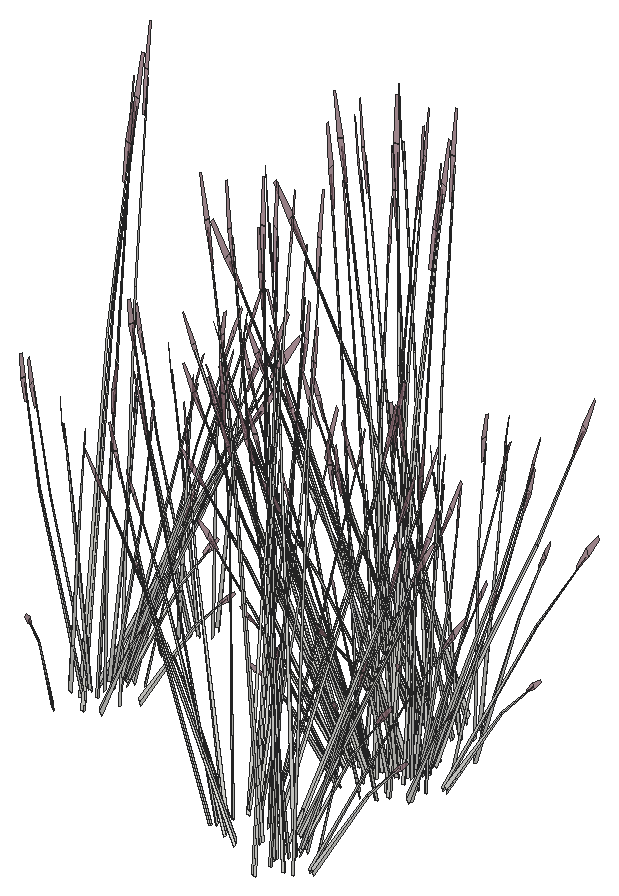
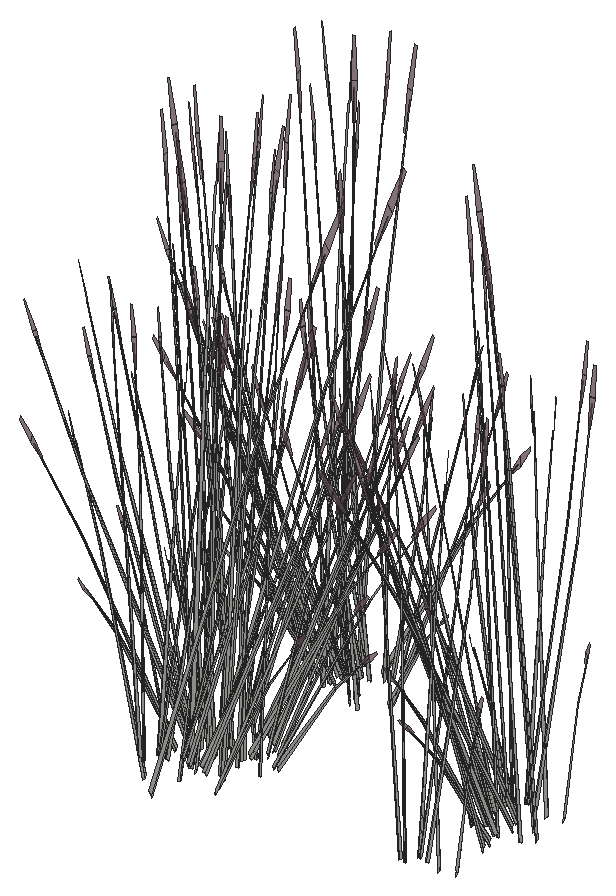
# SketchUp Ruby script. Lengths in inches.
U = 1.inch
M = Sketchup.active_model
def pt(a) = Geom::Point3d.new(a.map { |v| v * U })
def face(e, loops, mat)
  f = e.add_face(loops[0].map { |a| pt(a) })
  loops[1..].each { |l| e.add_face(l.map { |a| pt(a) }).erase! }
  f.material = f.back_material = mat if mat
  f
end
# faces: each face lists its corners as indices into pts; further lists are holes
def faces(e, pts, list, mat = nil) = list.each { |f| face(e, (f[0].is_a?(Array) ? f : [f]).map { |l| l.map { |i| pts[i] } }, mat) }
# xy, xz, yz: faces in a plane at the given z, y or x. An outline is a flat list of corners, or four numbers for a rectangle; further outlines are holes
def ring(l) = l.size == 4 ? [[l[0], l[1]], [l[2], l[1]], [l[2], l[3]], [l[0], l[3]]] : l.each_slice(2).to_a
def flat(e, list, mat, &to3) = list.each { |f| face(e, (f[0].is_a?(Array) ? f : [f]).map { |l| ring(l).map { |u, v| to3.(u, v) } }, mat) }
def xy(e, z, list, mat = nil) = flat(e, list, mat) { |x, y| [x, y, z] }
def xz(e, y, list, mat = nil) = flat(e, list, mat) { |x, z| [x, y, z] }
def yz(e, x, list, mat = nil) = flat(e, list, mat) { |y, z| [x, y, z] }
def lines(e, pts, list) = list.each { |a, b| e.add_line(pt(pts[a]), pt(pts[b])) }
# prism: a flat outline (further loops are holes) pulled along v
def prism(e, loops, v, mat = nil)
  f = face(e, loops, mat); d = Geom::Vector3d.new(v.map { |x| x * U })
  f.pushpull(f.normal.samedirection?(d) ? d.length : -d.length)
end
def box(e, o, s, mat = nil) = prism(e, [[o, [o[0] + s[0], o[1], o[2]], [o[0] + s[0], o[1] + s[1], o[2]], [o[0], o[1] + s[1], o[2]]]], [0, 0, s[2]], mat)
def at(x, y, z, deg = 0) = Geom::Transformation.translation(pt([x, y, z])) * Geom::Transformation.rotation(ORIGIN, Z_AXIS, deg.degrees)
def axes(o, x, y, z) = Geom::Transformation.new([*x, 0, *y, 0, *z, 0, *pt(o).to_a, 1])
def part(name) = M.definitions.add(name)
# library, detail: a bought-in or finely detailed component or shape, given as its bounding box
def library(name, o, s) = part(name).tap { |d| box(d.entities, o, s) }
def detail(e, o, s) = box(e.add_group.entities, o, s)
def put(e, d, t, mat = nil) = e.add_instance(d, t).tap { |i| i.material = mat if mat }
def group(e, t, mat = nil) = e.add_group.tap { |g| g.transformation = t; g.material = mat if mat }.entities
root = M.entities
M.materials.add("LightPink_Translucent").color = [144, 107, 117]
M.materials["LightPink_Translucent"].alpha = 0.75
c1 = part("blade")
p = [[2.15,0.21,22],[0,0.17,0],[0.09,0.45,0],[2.18,0.31,22],[2.29,0.31,22],[0.38,0.45,0],
  [2.48,0.24,33],[2.49,0.24,33],[2.48,0.22,33]]
faces(c1.entities,p,[[0,1,2,3],[4,5,2,3],[6,3,4,7],[8,0,3,6]])
c2 = part("seeds")
p = [[0.3,-0.1,1.38],[-0.01,-0.03,1.59],[-0.01,-0.03,0.03],[0.14,-0.07,-0.07],[0.29,-0.03,3],[0.15,0.01,3.11]]
faces(c2.entities,p,[[0,1,2,3],[1,0,4,5]],"LightPink_Translucent")
c3 = part("blade with seeds")
put(c3.entities,c1,at(0,0,0))
put(c3.entities,c2,axes([2.4,0.25,30.99],[1.5799,-0.05474,1.17369],[-0.12525,1.92788,0.29478],[-0.07173,-0.02425,1.56792]))
put(root,c3,axes([702.48,323.1875,513.76],[0.54068,0.15928,-0.29394],[-0.1577,0.46469,0.37948],[0.21769,-0.04261,0.72609]))
put(root,c3,axes([696.13,322.45,513.76],[-0.54068,-0.15928,-0.29394],[0.1577,-0.46469,0.37948],[-0.21769,0.04261,0.72609]))
put(root,c3,axes([700.58,321.42,512.05],[-0.6991,0.15154,0.14643],[-0.17263,-0.56398,0.29122],[0.06235,0.08217,1.33138]))
put(root,c3,axes([700.51,324.35,512.05],[0.18794,-0.56744,0.14643],[0.68774,0.16058,0.29122],[-0.1188,0.00276,1.33138]))
put(root,c3,axes([697.78,322.37,512.77],[0.18493,-0.0826,1.46963],[0.06377,0.5767,0.11501],[-0.40056,0.07652,0.52526]))
put(root,c3,axes([701.59,322.9,512.05],[-0.51116,-0.4159,0.14643],[0.51512,-0.4034,0.29122],[-0.05645,0.08494,1.33138]))
put(root,c3,axes([703.63,323.28,512.3],[-0.40197,0.09426,0.95334],[0.18921,-0.38956,0.70045],[0.21325,0.02666,0.20998]))
put(root,c3,axes([698.21,324.61,512.06],[0.60889,0.28548,0.4121],[-0.36394,0.51192,0],[-0.13868,-0.06502,1.30728]))
put(root,c3,axes([700.35,322.63,512.26],[0.31565,-0.51449,0.37133],[0.65588,0.24761,-0.17871],[0,0.1186,1.19224]))
put(root,c3,axes([696.5,322.6875,513.89],[-0.17625,0.51936,-0.42412],[-0.60429,-0.17802,-0.32852],[-0.2433,0.04762,0.81151]))
put(root,c3,axes([702.93,324.48,513.26],[-0.12452,-0.47997,-0.02898],[0.58854,-0.11034,-0.1314],[0.1229,0.03043,0.43341]))
put(root,c3,axes([702.01,322.92,512.06],[0,-0.57097,0.4121],[0.72788,0,0],[0,0.13004,1.30728]))
put(root,c3,axes([700.18,323.35,512.26],[0.70648,-0.03525,0.37133],[0.06389,0.58508,-0.17871],[-0.12647,0.0593,1.19224]))
put(root,c3,axes([702.88,323.91,512.15],[-0.15668,-0.14043,1.18691],[0.20386,-0.46454,-0.25526],[0.31701,0.06293,0.50747]))
put(root,c3,axes([701.44,324.19,514.13],[0.65035,0.01375,-0.58968],[-0.04368,0.5789,0.07116],[0.27552,0.06109,0.83415]))
put(root,c3,axes([700.71,324.65,512.06],[0.60889,-0.28548,0.4121],[0.36394,0.51192,0],[-0.13868,0.06502,1.30728]))
put(root,c3,axes([695.78,323.9,512.15],[0.2261,0.04687,1.18691],[0.14573,0.47875,-0.25526],[-0.30712,0.08962,0.50747]))
put(root,c3,axes([695.3,324.91,512.3],[0.27113,-0.25877,0.95334],[0.10699,0.40966,0.70045],[-0.19594,0.07335,0.20998]))
put(root,c3,axes([701.83,324.43,513.76],[0.37017,0.35748,-0.29394],[-0.42268,0.3384,0.37948],[0.21476,0.05149,0.72609]))
put(root,c3,axes([696.33,323.79,513.76],[-0.56631,0.0816,-0.29394],[-0.14954,-0.46647,0.37948],[-0.16229,0.12529,0.72609]))
put(root,c3,axes([678.84,331.31,514.13],[0.01693,-0.52814,-0.58968],[0.71285,0.03547,0.07116],[0.07523,-0.22375,0.83415]))
put(root,c3,axes([678.03,331.04,513.22],[-0.12114,0.19625,1.42242],[-0.50818,-0.40613,0.11501],[0.22925,-0.25313,0.60807]))
put(root,c3,axes([677.71,329.53,512.3],[0.08346,0.33295,0.95334],[-0.46298,-0.1844,0.70045],[0.04982,-0.17048,0.20998]))
put(root,c3,axes([701.4,324.63,512.3],[-0.36631,-0.16417,0.95334],[0.47299,-0.16681,0.70045],[0.12758,0.1413,0.20998]))
put(root,c3,axes([678.69,331.13,513.89],[-0.46573,-0.38364,-0.42412],[0.49199,-0.33598,-0.32852],[0.07086,-0.19492,0.81151]))
put(root,c3,axes([696.79,323.84,513.89],[0.16713,0.52135,-0.42412],[-0.63294,0.0912,-0.32852],[-0.18138,0.14003,0.81151]))
put(root,c3,axes([700.5,322.79,512.36],[-0.01777,-0.53759,1.17256],[0.80434,0.13935,0.49647],[-0.19024,0.29416,1.1068]))
put(root,c3,axes([700.57,324.86,513.89],[0.64198,-0.13573,-0.42412],[0.1123,0.514,-0.32852],[0.17243,0.1473,0.81151]))
put(root,c3,axes([679.13,330.99,513.76],[0.4402,-0.30062,-0.29394],[0.41671,0.34326,0.37948],[0.0634,-0.1744,0.72609]))
put(root,c3,axes([701.45,325.38,512.21],[-0.4172,-0.01791,0.872],[0.27552,-0.38032,0.48145],[0.16481,0.13512,0.68401]))
put(root,c3,axes([700.09,324.46,512.15],[0.01148,-0.18927,1.18691],[0.54864,-0.21141,-0.25526],[0.16937,0.22654,0.50747]))
put(root,c3,axes([697.32,324.87,513.76],[-0.4402,0.30062,-0.29394],[-0.41671,-0.34326,0.37948],[-0.0634,0.1744,0.72609]))
put(root,c3,axes([697.6,326.04,512.3],[-0.01684,-0.3395,0.95334],[0.42072,0.24214,0.70045],[-0.08274,0.16182,0.20998]))
put(root,c3,axes([679.68,332.23,514.13],[0.33983,-0.45051,-0.58968],[0.59551,0.32017,0.07116],[0.20291,-0.16322,0.83415]))
put(root,c3,axes([679.66,332.02,513.89],[-0.16713,-0.52135,-0.42412],[0.63294,-0.0912,-0.32852],[0.18138,-0.14003,0.81151]))
put(root,c3,axes([697.76,324.73,514.15],[0.46573,0.38364,-0.47077],[-0.49199,0.33598,-0.36465],[-0.07086,0.19492,0.90078]))
put(root,c3,axes([699.14,325.1,513.89],[0.63954,0.14313,-0.42412],[-0.21921,0.49074,-0.32852],[0.05864,0.19758,0.81151]))
put(root,c3,axes([698.85,325.4,513.76],[-0.19614,0.43908,-0.29394],[-0.57222,-0.12807,0.37948],[0.05247,0.17678,0.72609]))
put(root,c3,axes([700.55,333.73,512.15],[-0.18493,0.11557,1.18691],[-0.55384,-0.20228,-0.25526],[0.10266,-0.25157,0.50747]))
put(root,c3,axes([699.7,334.13,514.13],[-0.31051,-0.46426,-0.58968],[0.63919,-0.25873,0.07116],[-0.07261,-0.22432,0.83415]))
put(root,c3,axes([697.62,324.55,514.43],[-0.01693,0.52814,-0.65454],[-0.71285,-0.03547,0.07899],[-0.07523,0.22375,0.92591]))
put(root,c3,axes([697.68,333.51,512.15],[-0.0394,0.18678,1.18691],[-0.57594,0.15636,-0.25526],[-0.13463,-0.24142,0.50747]))
put(root,c3,axes([680.4375,330.98,512.3],[-0.2167,0.29065,0.95334],[-0.18626,-0.3905,0.70045],[0.17898,-0.09785,0.20998]))
put(root,c3,axes([701,334.59,514.13],[0.01693,-0.52814,-0.58968],[0.71285,0.03547,0.07116],[0.07523,-0.22375,0.83415]))
put(root,c3,axes([680.125,332.07,513.76],[0.56631,-0.0816,-0.29394],[0.14954,0.46647,0.37948],[0.16229,-0.12529,0.72609]))
put(root,c3,axes([698.91,325,514.13],[0.31051,0.46426,-0.58968],[-0.63919,0.25873,0.07116],[0.07261,0.22432,0.83415]))
put(root,c3,axes([697.11,325.74,512.15],[0.2053,-0.09007,1.18691],[0.50689,0.27159,-0.25526],[-0.15087,0.235,0.50747]))
put(root,c3,axes([699.76,333.74,513.76],[0.19614,-0.43908,-0.29394],[0.57222,0.12807,0.37948],[-0.05247,-0.17678,0.72609]))
put(root,c3,axes([699.47,334.04,513.89],[-0.63954,-0.14313,-0.42412],[0.21921,-0.49074,-0.32852],[-0.05864,-0.19758,0.81151]))
put(root,c3,axes([699.87,332.81,512.3],[0.08346,0.33295,0.95334],[-0.46298,-0.1844,0.70045],[0.04982,-0.17048,0.20998]))
put(root,c3,axes([700.85,334.41,513.89],[-0.46573,-0.38364,-0.42412],[0.49199,-0.33598,-0.32852],[0.07086,-0.19492,0.81151]))
put(root,c3,axes([697.38,325.29,512.79],[0.01429,-0.29475,1.28107],[0.64291,0.15569,0.17703],[-0.0557,0.31414,0.60492]))
put(root,c3,axes([701.29,334.27,513.76],[0.4402,-0.30062,-0.29394],[0.41671,0.34326,0.37948],[0.0634,-0.1744,0.72609]))
put(root,c3,axes([697.49,333.21,512.3],[0.33937,0.19872,0.95334],[-0.49424,0.11946,0.70045],[-0.10575,-0.15273,0.20998]))
put(root,c3,axes([698.3,334.26,514.13],[-0.55475,-0.27598,-0.58968],[0.39425,-0.48361,0.07116],[-0.20099,-0.16478,0.83415]))
put(root,c3,axes([698.11,333.9,513.76],[-0.10048,-0.4599,-0.29394],[0.5744,-0.12144,0.37948],[-0.15428,-0.13179,0.72609]))
put(root,c3,axes([679.95,333.18,513.89],[0.17625,-0.51936,-0.42412],[0.60429,0.17802,-0.32852],[0.2433,-0.04762,0.81151]))
put(root,c3,axes([698.05,334.28,513.89],[-0.64198,0.13573,-0.42412],[-0.1123,-0.514,-0.32852],[-0.17243,-0.1473,0.81151]))
put(root,c3,axes([701.84,335.5,514.13],[0.33983,-0.45051,-0.58968],[0.59551,0.32017,0.07116],[0.20291,-0.16322,0.83415]))
put(root,c3,axes([701.82,335.29,513.89],[-0.16713,-0.52135,-0.42412],[0.63294,-0.0912,-0.32852],[0.18138,-0.14003,0.81151]))
put(root,c3,axes([678.65,331.36,512.06],[-0.60889,-0.28548,0.4121],[0.36394,-0.51192,0],[0.13868,0.06502,1.30728]))
put(root,c3,axes([679.84,333.36,514.13],[0.57168,-0.25217,-0.58968],[0.3186,0.51908,0.07116],[0.27622,-0.05897,0.83415]))
put(root,c3,axes([699.63,337.39,512.76],[0.56221,0.23024,1.25546],[-0.55078,0.49601,0.49647],[-0.2467,-0.29398,1.05249]))
put(root,c3,axes([702.33,335.09,512.15],[-0.23242,-0.01691,1.18691],[-0.23811,-0.45367,-0.25526],[0.28553,-0.12834,0.50747]))
put(root,c3,axes([677.51,332.38,512.26],[-0.39083,-0.47924,0.37133],[0.59199,-0.33747,-0.17871],[0.12647,0.0593,1.19224]))
put(root,c3,axes([702.6,334.26,512.3],[-0.2167,0.29065,0.95334],[-0.18626,-0.3905,0.70045],[0.17898,-0.09785,0.20998]))
put(root,c3,axes([680.32,333.41,513.76],[0.54068,0.15928,-0.29394],[-0.1577,0.46469,0.37948],[0.21769,-0.04261,0.72609]))
put(root,c3,axes([702.29,335.35,513.76],[0.56631,-0.0816,-0.29394],[0.14954,0.46647,0.37948],[0.16229,-0.12529,0.72609]))
put(root,c3,axes([696.78,334.71,513.76],[-0.37017,-0.35748,-0.29394],[0.42268,-0.3384,0.37948],[-0.21476,-0.05149,0.72609]))
put(root,c3,axes([678.85,332.84,513.22],[-0.26985,0.01293,1.42242],[0.17902,-0.56047,0.11501],[0.38456,0.03467,0.60807]))
put(root,c3,axes([696.65,335.09,512.15],[0.12702,0.15896,1.18691],[-0.2927,0.4321,-0.25526],[-0.30054,-0.10328,0.50747]))
put(root,c3,axes([697.17,334.95,514.13],[-0.65035,-0.01375,-0.58968],[0.04368,-0.5789,0.07116],[-0.27552,-0.06109,0.83415]))
put(root,c3,axes([681.47,333.51,512.3],[-0.40197,0.09426,0.95334],[0.18921,-0.38956,0.70045],[0.21325,0.02666,0.20998]))
put(root,c3,axes([678.19,332.86,512.26],[0.31565,-0.51449,0.37133],[0.65588,0.24761,-0.17871],[0,0.1186,1.19224]))
put(root,c3,axes([696.96,335.0625,513.89],[-0.47241,0.37822,-0.42412],[-0.41372,-0.39954,-0.32852],[-0.24002,-0.05755,0.81151]))
put(root,c3,axes([680.77,334.71,513.26],[-0.12452,-0.47997,-0.02898],[0.58854,-0.11034,-0.1314],[0.1229,0.03043,0.43341]))
put(root,c3,axes([695.89,335.56,512.3],[0.41536,-0.04086,0.95334],[-0.26347,0.35999,0.70045],[-0.20525,-0.054,0.20998]))
put(root,c3,axes([679.85,333.14,512.06],[0,-0.57097,0.4121],[0.72788,0,0],[0,0.13004,1.30728]))
put(root,c3,axes([698.83,335.9,512.26],[-0.70648,0.03525,0.37133],[-0.06389,-0.58508,-0.17871],[0.12647,-0.0593,1.19224]))
put(root,c3,axes([697.01,336.32,512.06],[0,0.57097,0.4121],[-0.72788,0,0],[0,-0.13004,1.30728]))
put(root,c3,axes([702.11,336.45,513.89],[0.17625,-0.51936,-0.42412],[0.60429,0.17802,-0.32852],[0.2433,-0.04762,0.81151]))
put(root,c3,axes([698.66,336.61,512.26],[-0.31565,0.51449,0.37133],[-0.65588,-0.24761,-0.17871],[0,-0.1186,1.19224]))
put(root,c3,axes([700.81,334.64,512.06],[-0.60889,-0.28548,0.4121],[0.36394,-0.51192,0],[0.13868,0.06502,1.30728]))
put(root,c3,axes([702,336.64,514.13],[0.57168,-0.25217,-0.58968],[0.3186,0.51908,0.07116],[0.27622,-0.05897,0.83415]))
put(root,c3,axes([698.5,334.89,512.05],[-0.18794,0.56744,0.14643],[-0.68774,-0.16058,0.29122],[0.1188,-0.00276,1.33138]))
put(root,c3,axes([679.28,334.41,514.13],[0.65035,0.01375,-0.58968],[-0.04368,0.5789,0.07116],[0.27552,0.06109,0.83415]))
put(root,c3,axes([700.55,340.13,512.15],[-0.18493,0.11557,1.18691],[-0.55384,-0.20228,-0.25526],[0.10266,-0.25157,0.50747]))
put(root,c3,axes([699.7,340.53,514.13],[-0.31051,-0.46426,-0.58968],[0.63919,-0.25873,0.07116],[-0.07261,-0.22432,0.83415]))
put(root,c3,axes([697.68,339.91,512.15],[-0.0394,0.18678,1.18691],[-0.57594,0.15636,-0.25526],[-0.13463,-0.24142,0.50747]))
put(root,c3,axes([699.67,335.66,512.26],[-0.39083,-0.47924,0.37133],[0.59199,-0.33747,-0.17871],[0.12647,0.0593,1.19224]))
put(root,c3,axes([679.67,334.65,513.76],[0.37017,0.35748,-0.29394],[-0.42268,0.3384,0.37948],[0.21476,0.05149,0.72609]))
put(root,c3,axes([679.82,340.99,514.13],[0.01693,-0.52814,-0.58968],[0.71285,0.03547,0.07116],[0.07523,-0.22375,0.83415]))
put(root,c3,axes([701,340.99,514.13],[0.01693,-0.52814,-0.58968],[0.71285,0.03547,0.07116],[0.07523,-0.22375,0.83415]))
put(root,c3,axes([698.43,337.82,512.05],[0.6991,-0.15154,0.14643],[0.17263,0.56398,0.29122],[-0.06235,-0.08217,1.33138]))
put(root,c3,axes([702.48,336.6875,513.76],[0.54068,0.15928,-0.29394],[-0.1577,0.46469,0.37948],[0.21769,-0.04261,0.72609]))
put(root,c3,axes([699.76,340.14,513.76],[0.19614,-0.43908,-0.29394],[0.57222,0.12807,0.37948],[-0.05247,-0.17678,0.72609]))
put(root,c3,axes([679.02,340.72,513.22],[-0.12114,0.19625,1.42242],[-0.50818,-0.40613,0.11501],[0.22925,-0.25313,0.60807]))
put(root,c3,axes([696.13,335.95,513.76],[-0.54068,-0.15928,-0.29394],[0.1577,-0.46469,0.37948],[-0.21769,0.04261,0.72609]))
put(root,c3,axes([700.58,334.92,512.05],[-0.6991,0.15154,0.14643],[-0.17263,-0.56398,0.29122],[0.06235,0.08217,1.33138]))
put(root,c3,axes([699.47,340.4375,513.89],[-0.63954,-0.14313,-0.42412],[0.21921,-0.49074,-0.32852],[-0.05864,-0.19758,0.81151]))
put(root,c3,axes([678.69,339.21,512.3],[0.08346,0.33295,0.95334],[-0.46298,-0.1844,0.70045],[0.04982,-0.17048,0.20998]))
put(root,c3,axes([699.87,339.21,512.3],[0.08346,0.33295,0.95334],[-0.46298,-0.1844,0.70045],[0.04982,-0.17048,0.20998]))
put(root,c3,axes([679.68,340.8125,513.89],[-0.46573,-0.38364,-0.42412],[0.49199,-0.33598,-0.32852],[0.07086,-0.19492,0.81151]))
put(root,c3,axes([700.85,340.8125,513.89],[-0.46573,-0.38364,-0.42412],[0.49199,-0.33598,-0.32852],[0.07086,-0.19492,0.81151]))
put(root,c3,axes([678.34,333.74,513.22],[-0.24166,-0.09837,1.42242],[0.50011,-0.41269,0.11501],[0.3117,0.18617,0.60807]))
put(root,c3,axes([700.51,337.85,512.05],[0.18794,-0.56744,0.14643],[0.68774,0.16058,0.29122],[-0.1188,0.00276,1.33138]))
put(root,c3,axes([679.24,334.86,512.3],[-0.36631,-0.16417,0.95334],[0.47299,-0.16681,0.70045],[0.12758,0.1413,0.20998]))
put(root,c3,axes([680.12,340.67,513.76],[0.4402,-0.30062,-0.29394],[0.41671,0.34326,0.37948],[0.0634,-0.1744,0.72609]))
put(root,c3,axes([701.29,340.67,513.76],[0.4402,-0.30062,-0.29394],[0.41671,0.34326,0.37948],[0.0634,-0.1744,0.72609]))
put(root,c3,axes([697.49,339.61,512.3],[0.33937,0.19872,0.95334],[-0.49424,0.11946,0.70045],[-0.10575,-0.15273,0.20998]))
put(root,c3,axes([698.3,340.66,514.13],[-0.55475,-0.27598,-0.58968],[0.39425,-0.48361,0.07116],[-0.20099,-0.16478,0.83415]))
put(root,c3,axes([698.11,340.3,513.76],[-0.10048,-0.4599,-0.29394],[0.5744,-0.12144,0.37948],[-0.15428,-0.13179,0.72609]))
put(root,c3,axes([697.78,335.87,512.77],[0.18493,-0.0826,1.46963],[0.06377,0.5767,0.11501],[-0.40056,0.07652,0.52526]))
put(root,c3,axes([701.59,336.4,512.05],[-0.51116,-0.4159,0.14643],[0.51512,-0.4034,0.29122],[-0.05645,0.08494,1.33138]))
put(root,c3,axes([703.63,336.78,512.3],[-0.40197,0.09426,0.95334],[0.18921,-0.38956,0.70045],[0.21325,0.02666,0.20998]))
put(root,c3,axes([698.21,338.11,512.06],[0.60889,0.28548,0.4121],[-0.36394,0.51192,0],[-0.13868,-0.06502,1.30728]))
put(root,c3,axes([700.35,336.13,512.26],[0.31565,-0.51449,0.37133],[0.65588,0.24761,-0.17871],[0,0.1186,1.19224]))
put(root,c3,axes([678.41,335.08,513.89],[0.64198,-0.13573,-0.42412],[0.1123,0.514,-0.32852],[0.17243,0.1473,0.81151]))
put(root,c3,axes([696.5,336.1875,513.89],[-0.17625,0.51936,-0.42412],[-0.60429,-0.17802,-0.32852],[-0.2433,0.04762,0.81151]))
put(root,c3,axes([702.93,337.98,513.26],[-0.12452,-0.47997,-0.02898],[0.58854,-0.11034,-0.1314],[0.1229,0.03043,0.43341]))
put(root,c3,axes([679.29,335.6,512.21],[-0.4172,-0.01791,0.872],[0.27552,-0.38032,0.48145],[0.16481,0.13512,0.68401]))
put(root,c3,axes([702.01,336.42,512.06],[0,-0.57097,0.4121],[0.72788,0,0],[0,0.13004,1.30728]))
put(root,c3,axes([700.18,336.85,512.26],[0.70648,-0.03525,0.37133],[0.06389,0.58508,-0.17871],[-0.12647,0.0593,1.19224]))
put(root,c3,axes([698.05,340.68,513.89],[-0.64198,0.13573,-0.42412],[-0.1123,-0.514,-0.32852],[-0.17243,-0.1473,0.81151]))
put(root,c3,axes([702.88,337.41,512.15],[-0.15668,-0.14043,1.18691],[0.20386,-0.46454,-0.25526],[0.31701,0.06293,0.50747]))
put(root,c3,axes([680.66,341.9,514.13],[0.33983,-0.45051,-0.58968],[0.59551,0.32017,0.07116],[0.20291,-0.16322,0.83415]))
put(root,c3,axes([701.84,341.9,514.13],[0.33983,-0.45051,-0.58968],[0.59551,0.32017,0.07116],[0.20291,-0.16322,0.83415]))
put(root,c3,axes([680.65,341.69,513.89],[-0.16713,-0.52135,-0.42412],[0.63294,-0.0912,-0.32852],[0.18138,-0.14003,0.81151]))
put(root,c3,axes([701.82,341.69,513.89],[-0.16713,-0.52135,-0.42412],[0.63294,-0.0912,-0.32852],[0.18138,-0.14003,0.81151]))
put(root,c3,axes([699.63,343.79,512.76],[0.56221,0.23024,1.25546],[-0.55078,0.49601,0.49647],[-0.2467,-0.29398,1.05249]))
put(root,c3,axes([701.44,337.69,514.13],[0.65035,0.01375,-0.58968],[-0.04368,0.5789,0.07116],[0.27552,0.06109,0.83415]))
put(root,c3,axes([700.71,338.15,512.06],[0.60889,-0.28548,0.4121],[0.36394,0.51192,0],[-0.13868,0.06502,1.30728]))
put(root,c3,axes([702.33,341.49,512.15],[-0.23242,-0.01691,1.18691],[-0.23811,-0.45367,-0.25526],[0.28553,-0.12834,0.50747]))
